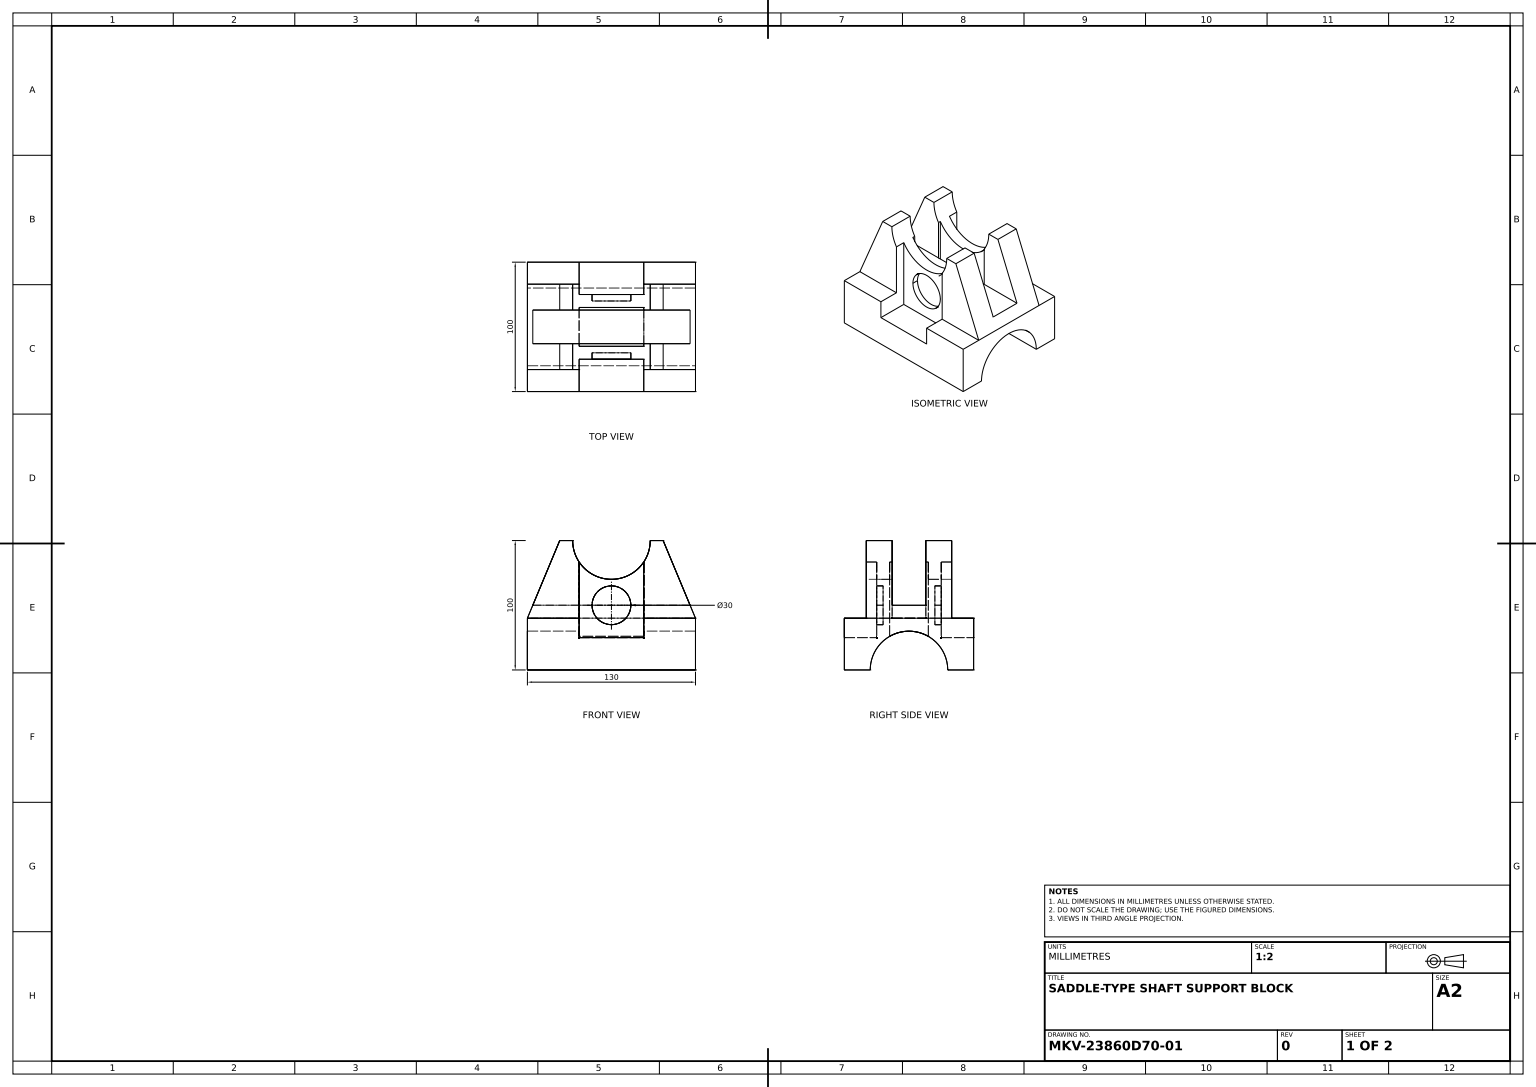
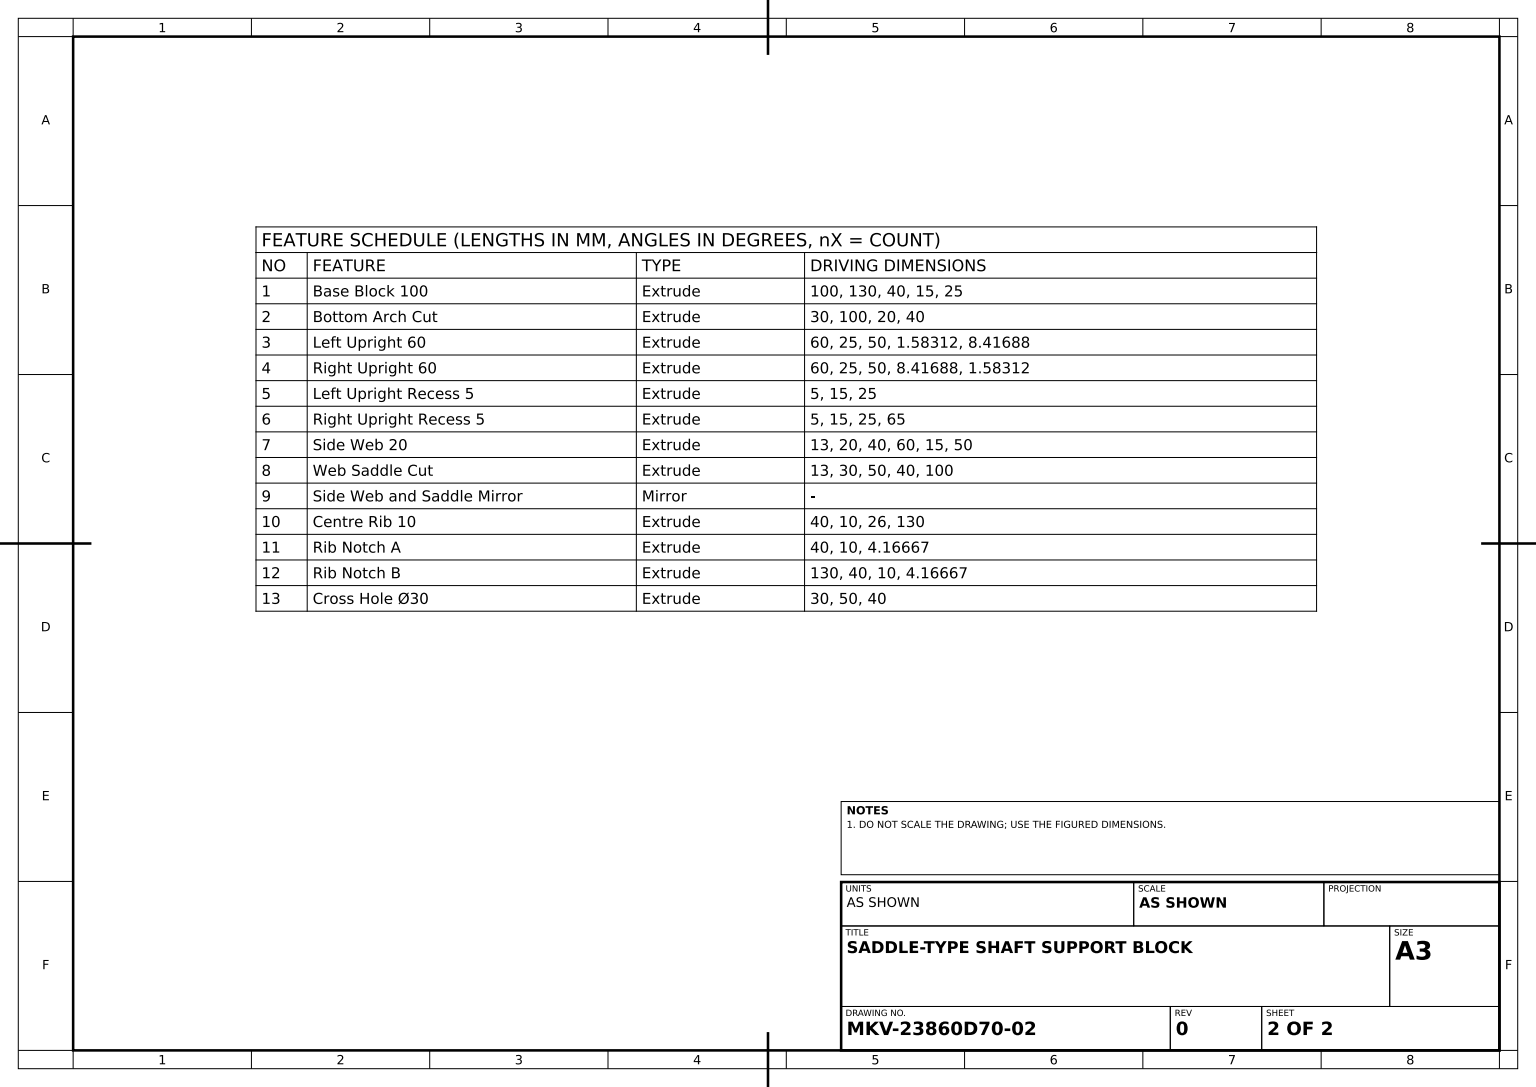
ISO-10303-21;
HEADER;
FILE_DESCRIPTION((''),'2;1');
FILE_NAME('','',(''),(''),'','','');
FILE_SCHEMA(('AUTOMOTIVE_DESIGN'));
ENDSEC;
DATA;
#1=APPLICATION_CONTEXT('');
#2=PRODUCT_CONTEXT('',#1,'mechanical');
#3=PRODUCT('','','',(#2));
#4=PRODUCT_DEFINITION_FORMATION('','',#3);
#5=PRODUCT_DEFINITION_CONTEXT('',#1,'design');
#6=PRODUCT_DEFINITION('','',#4,#5);
#7=PRODUCT_DEFINITION_SHAPE('','',#6);
#8=(LENGTH_UNIT()NAMED_UNIT(*)SI_UNIT(.MILLI.,.METRE.));
#9=(NAMED_UNIT(*)PLANE_ANGLE_UNIT()SI_UNIT($,.RADIAN.));
#10=(NAMED_UNIT(*)SI_UNIT($,.STERADIAN.)SOLID_ANGLE_UNIT());
#11=UNCERTAINTY_MEASURE_WITH_UNIT(LENGTH_MEASURE(1.E-05),#8,'distance_accuracy_value','');
#12=(GEOMETRIC_REPRESENTATION_CONTEXT(3)GLOBAL_UNCERTAINTY_ASSIGNED_CONTEXT((#11))GLOBAL_UNIT_ASSIGNED_CONTEXT((#8,#9,#10))REPRESENTATION_CONTEXT('',''));
#13=CARTESIAN_POINT('',(90.,40.,-33.));
#14=VERTEX_POINT('',#13);
#15=CARTESIAN_POINT('',(90.,40.,-50.));
#16=VERTEX_POINT('',#15);
#17=CARTESIAN_POINT('',(90.,40.,50.));
#18=DIRECTION('',(0.,0.,-1.));
#19=VECTOR('',#18,1000.);
#20=LINE('',#17,#19);
#21=EDGE_CURVE('',#14,#16,#20,.T.);
#22=ORIENTED_EDGE('',*,*,#21,.F.);
#23=CARTESIAN_POINT('',(130.,40.,-33.));
#24=VERTEX_POINT('',#23);
#25=DIRECTION('',(1.,0.,0.));
#26=VECTOR('',#25,1000.);
#27=LINE('',#23,#26);
#28=EDGE_CURVE('',#14,#24,#27,.T.);
#29=ORIENTED_EDGE('',*,*,#28,.T.);
#30=CARTESIAN_POINT('',(130.,40.,-50.));
#31=VERTEX_POINT('',#30);
#32=CARTESIAN_POINT('',(130.,40.,50.));
#33=LINE('',#32,#19);
#34=EDGE_CURVE('',#24,#31,#33,.T.);
#35=ORIENTED_EDGE('',*,*,#34,.T.);
#36=CARTESIAN_POINT('',(0.,40.,-50.));
#37=DIRECTION('',(-1.,0.,0.));
#38=VECTOR('',#37,1000.);
#39=LINE('',#36,#38);
#40=EDGE_CURVE('',#31,#16,#39,.T.);
#41=ORIENTED_EDGE('',*,*,#40,.T.);
#42=EDGE_LOOP('',(#22,#29,#35,#41));
#43=FACE_OUTER_BOUND('',#42,.T.);
#44=CARTESIAN_POINT('',(0.,40.,50.));
#45=DIRECTION('',(0.,-1.,0.));
#46=AXIS2_PLACEMENT_3D('',#44,#45,#18);
#47=PLANE('',#46);
#48=ADVANCED_FACE('',(#43),#47,.F.);
#49=CARTESIAN_POINT('',(40.,83.416876,-15.));
#50=VERTEX_POINT('',#49);
#51=CARTESIAN_POINT('',(40.,25.980762,-15.));
#52=VERTEX_POINT('',#51);
#53=CARTESIAN_POINT('',(40.,85.,-15.));
#54=VECTOR('',#45,1000.);
#55=LINE('',#53,#54);
#56=EDGE_CURVE('',#50,#52,#55,.T.);
#57=ORIENTED_EDGE('',*,*,#56,.T.);
#58=CARTESIAN_POINT('',(90.,25.980762,-15.));
#59=VERTEX_POINT('',#58);
#60=CARTESIAN_POINT('',(0.,25.980762,-15.));
#61=LINE('',#60,#38);
#62=EDGE_CURVE('',#59,#52,#61,.T.);
#63=ORIENTED_EDGE('',*,*,#62,.F.);
#64=CARTESIAN_POINT('',(90.,83.416876,-15.));
#65=VERTEX_POINT('',#64);
#66=CARTESIAN_POINT('',(90.,85.,-15.));
#67=LINE('',#66,#54);
#68=EDGE_CURVE('',#65,#59,#67,.T.);
#69=ORIENTED_EDGE('',*,*,#68,.F.);
#70=CARTESIAN_POINT('',(65.,100.,-15.));
#71=DIRECTION('',(0.,0.,1.));
#72=AXIS2_PLACEMENT_3D('',#70,#71,#25);
#73=CIRCLE('',#72,30.);
#74=EDGE_CURVE('',#50,#65,#73,.T.);
#75=ORIENTED_EDGE('',*,*,#74,.F.);
#76=EDGE_LOOP('',(#57,#63,#69,#75));
#77=FACE_OUTER_BOUND('',#76,.T.);
#78=AXIS2_PLACEMENT_3D('',#66,#71,#25);
#79=PLANE('',#78);
#80=ADVANCED_FACE('',(#77),#79,.T.);
#81=CARTESIAN_POINT('',(50.,50.,25.));
#82=VERTEX_POINT('',#81);
#83=CARTESIAN_POINT('',(80.,50.,25.));
#84=VERTEX_POINT('',#83);
#85=CARTESIAN_POINT('',(65.,50.,25.));
#86=AXIS2_PLACEMENT_3D('',#85,#71,#25);
#87=CIRCLE('',#86,15.);
#88=EDGE_CURVE('',#82,#84,#87,.T.);
#89=ORIENTED_EDGE('',*,*,#88,.T.);
#90=CARTESIAN_POINT('',(80.,50.,20.));
#91=VERTEX_POINT('',#90);
#92=VECTOR('',#71,1000.);
#93=LINE('',#90,#92);
#94=EDGE_CURVE('',#91,#84,#93,.T.);
#95=ORIENTED_EDGE('',*,*,#94,.F.);
#96=CARTESIAN_POINT('',(50.,50.,20.));
#97=VERTEX_POINT('',#96);
#98=CARTESIAN_POINT('',(65.,50.,20.));
#99=AXIS2_PLACEMENT_3D('',#98,#71,#25);
#100=CIRCLE('',#99,15.);
#101=EDGE_CURVE('',#97,#91,#100,.T.);
#102=ORIENTED_EDGE('',*,*,#101,.F.);
#103=LINE('',#96,#92);
#104=EDGE_CURVE('',#97,#82,#103,.T.);
#105=ORIENTED_EDGE('',*,*,#104,.T.);
#106=EDGE_LOOP('',(#89,#95,#102,#105));
#107=FACE_OUTER_BOUND('',#106,.T.);
#108=CYLINDRICAL_SURFACE('',#99,15.);
#109=ADVANCED_FACE('',(#107),#108,.F.);
#110=CARTESIAN_POINT('',(90.,40.,13.));
#111=VERTEX_POINT('',#110);
#112=CARTESIAN_POINT('',(90.,40.,-13.));
#113=VERTEX_POINT('',#112);
#114=EDGE_CURVE('',#111,#113,#20,.T.);
#115=ORIENTED_EDGE('',*,*,#114,.F.);
#116=CARTESIAN_POINT('',(40.,40.,13.));
#117=VERTEX_POINT('',#116);
#118=CARTESIAN_POINT('',(0.,40.,13.));
#119=LINE('',#118,#26);
#120=EDGE_CURVE('',#117,#111,#119,.T.);
#121=ORIENTED_EDGE('',*,*,#120,.F.);
#122=CARTESIAN_POINT('',(40.,40.,-13.));
#123=VERTEX_POINT('',#122);
#124=CARTESIAN_POINT('',(40.,40.,50.));
#125=LINE('',#124,#19);
#126=EDGE_CURVE('',#117,#123,#125,.T.);
#127=ORIENTED_EDGE('',*,*,#126,.T.);
#128=CARTESIAN_POINT('',(130.,40.,-13.));
#129=LINE('',#128,#38);
#130=EDGE_CURVE('',#113,#123,#129,.T.);
#131=ORIENTED_EDGE('',*,*,#130,.F.);
#132=EDGE_LOOP('',(#115,#121,#127,#131));
#133=FACE_OUTER_BOUND('',#132,.T.);
#134=CARTESIAN_POINT('',(0.,40.,0.));
#135=DIRECTION('',(0.,1.,0.));
#136=AXIS2_PLACEMENT_3D('',#134,#135,#71);
#137=PLANE('',#136);
#138=ADVANCED_FACE('',(#133),#137,.F.);
#139=CARTESIAN_POINT('',(0.,40.,-33.));
#140=VERTEX_POINT('',#139);
#141=CARTESIAN_POINT('',(40.,40.,-33.));
#142=VERTEX_POINT('',#141);
#143=LINE('',#139,#26);
#144=EDGE_CURVE('',#140,#142,#143,.T.);
#145=ORIENTED_EDGE('',*,*,#144,.F.);
#146=CARTESIAN_POINT('',(25.,100.,-33.));
#147=VERTEX_POINT('',#146);
#148=DIRECTION('',(-0.384615385,-0.923076923,0.));
#149=VECTOR('',#148,1000.);
#150=LINE('',#146,#149);
#151=EDGE_CURVE('',#147,#140,#150,.T.);
#152=ORIENTED_EDGE('',*,*,#151,.F.);
#153=CARTESIAN_POINT('',(35.,100.,-33.));
#154=VERTEX_POINT('',#153);
#155=LINE('',#146,#38);
#156=EDGE_CURVE('',#154,#147,#155,.T.);
#157=ORIENTED_EDGE('',*,*,#156,.F.);
#158=CARTESIAN_POINT('',(40.,83.416876,-33.));
#159=VERTEX_POINT('',#158);
#160=CARTESIAN_POINT('',(65.,100.,-33.));
#161=AXIS2_PLACEMENT_3D('',#160,#71,#37);
#162=CIRCLE('',#161,30.);
#163=EDGE_CURVE('',#154,#159,#162,.T.);
#164=ORIENTED_EDGE('',*,*,#163,.T.);
#165=VECTOR('',#135,1000.);
#166=LINE('',#141,#165);
#167=EDGE_CURVE('',#142,#159,#166,.T.);
#168=ORIENTED_EDGE('',*,*,#167,.F.);
#169=EDGE_LOOP('',(#145,#152,#157,#164,#168));
#170=FACE_OUTER_BOUND('',#169,.T.);
#171=CARTESIAN_POINT('',(0.,0.,-33.));
#172=AXIS2_PLACEMENT_3D('',#171,#18,#25);
#173=PLANE('',#172);
#174=ADVANCED_FACE('',(#170),#173,.T.);
#175=CARTESIAN_POINT('',(80.,50.,-20.));
#176=VERTEX_POINT('',#175);
#177=CARTESIAN_POINT('',(50.,50.,-20.));
#178=VERTEX_POINT('',#177);
#179=CARTESIAN_POINT('',(65.,50.,-20.));
#180=AXIS2_PLACEMENT_3D('',#179,#18,#37);
#181=CIRCLE('',#180,15.);
#182=EDGE_CURVE('',#176,#178,#181,.T.);
#183=ORIENTED_EDGE('',*,*,#182,.F.);
#184=CARTESIAN_POINT('',(80.,50.,-25.));
#185=VERTEX_POINT('',#184);
#186=LINE('',#175,#19);
#187=EDGE_CURVE('',#176,#185,#186,.T.);
#188=ORIENTED_EDGE('',*,*,#187,.T.);
#189=CARTESIAN_POINT('',(50.,50.,-25.));
#190=VERTEX_POINT('',#189);
#191=CARTESIAN_POINT('',(65.,50.,-25.));
#192=AXIS2_PLACEMENT_3D('',#191,#18,#37);
#193=CIRCLE('',#192,15.);
#194=EDGE_CURVE('',#185,#190,#193,.T.);
#195=ORIENTED_EDGE('',*,*,#194,.T.);
#196=LINE('',#177,#19);
#197=EDGE_CURVE('',#178,#190,#196,.T.);
#198=ORIENTED_EDGE('',*,*,#197,.F.);
#199=EDGE_LOOP('',(#183,#188,#195,#198));
#200=FACE_OUTER_BOUND('',#199,.T.);
#201=CYLINDRICAL_SURFACE('',#180,15.);
#202=ADVANCED_FACE('',(#200),#201,.F.);
#203=CARTESIAN_POINT('',(35.,100.,33.));
#204=VERTEX_POINT('',#203);
#205=CARTESIAN_POINT('',(35.,100.,13.));
#206=VERTEX_POINT('',#205);
#207=CARTESIAN_POINT('',(35.,100.,-50.));
#208=LINE('',#207,#19);
#209=EDGE_CURVE('',#204,#206,#208,.T.);
#210=ORIENTED_EDGE('',*,*,#209,.F.);
#211=CARTESIAN_POINT('',(40.,83.416876,33.));
#212=VERTEX_POINT('',#211);
#213=CARTESIAN_POINT('',(65.,100.,33.));
#214=AXIS2_PLACEMENT_3D('',#213,#71,#25);
#215=CIRCLE('',#214,30.);
#216=EDGE_CURVE('',#204,#212,#215,.T.);
#217=ORIENTED_EDGE('',*,*,#216,.T.);
#218=CARTESIAN_POINT('',(40.,83.416876,25.));
#219=VERTEX_POINT('',#218);
#220=CARTESIAN_POINT('',(40.,83.416876,-50.));
#221=LINE('',#220,#92);
#222=EDGE_CURVE('',#219,#212,#221,.T.);
#223=ORIENTED_EDGE('',*,*,#222,.F.);
#224=CARTESIAN_POINT('',(90.,83.416876,25.));
#225=VERTEX_POINT('',#224);
#226=CARTESIAN_POINT('',(65.,100.,25.));
#227=AXIS2_PLACEMENT_3D('',#226,#18,#37);
#228=CIRCLE('',#227,30.);
#229=EDGE_CURVE('',#225,#219,#228,.T.);
#230=ORIENTED_EDGE('',*,*,#229,.F.);
#231=CARTESIAN_POINT('',(90.,83.416876,33.));
#232=VERTEX_POINT('',#231);
#233=CARTESIAN_POINT('',(90.,83.416876,-50.));
#234=LINE('',#233,#19);
#235=EDGE_CURVE('',#232,#225,#234,.T.);
#236=ORIENTED_EDGE('',*,*,#235,.F.);
#237=CARTESIAN_POINT('',(95.,100.,33.));
#238=VERTEX_POINT('',#237);
#239=AXIS2_PLACEMENT_3D('',#213,#18,#37);
#240=CIRCLE('',#239,30.);
#241=EDGE_CURVE('',#238,#232,#240,.T.);
#242=ORIENTED_EDGE('',*,*,#241,.F.);
#243=CARTESIAN_POINT('',(95.,100.,13.));
#244=VERTEX_POINT('',#243);
#245=CARTESIAN_POINT('',(95.,100.,-50.));
#246=LINE('',#245,#92);
#247=EDGE_CURVE('',#244,#238,#246,.T.);
#248=ORIENTED_EDGE('',*,*,#247,.F.);
#249=CARTESIAN_POINT('',(90.,83.416876,13.));
#250=VERTEX_POINT('',#249);
#251=CARTESIAN_POINT('',(65.,100.,13.));
#252=AXIS2_PLACEMENT_3D('',#251,#18,#37);
#253=CIRCLE('',#252,30.);
#254=EDGE_CURVE('',#244,#250,#253,.T.);
#255=ORIENTED_EDGE('',*,*,#254,.T.);
#256=CARTESIAN_POINT('',(90.,83.416876,15.));
#257=VERTEX_POINT('',#256);
#258=EDGE_CURVE('',#257,#250,#234,.T.);
#259=ORIENTED_EDGE('',*,*,#258,.F.);
#260=CARTESIAN_POINT('',(40.,83.416876,15.));
#261=VERTEX_POINT('',#260);
#262=CARTESIAN_POINT('',(65.,100.,15.));
#263=AXIS2_PLACEMENT_3D('',#262,#71,#25);
#264=CIRCLE('',#263,30.);
#265=EDGE_CURVE('',#261,#257,#264,.T.);
#266=ORIENTED_EDGE('',*,*,#265,.F.);
#267=CARTESIAN_POINT('',(40.,83.416876,13.));
#268=VERTEX_POINT('',#267);
#269=EDGE_CURVE('',#268,#261,#221,.T.);
#270=ORIENTED_EDGE('',*,*,#269,.F.);
#271=AXIS2_PLACEMENT_3D('',#251,#71,#25);
#272=CIRCLE('',#271,30.);
#273=EDGE_CURVE('',#206,#268,#272,.T.);
#274=ORIENTED_EDGE('',*,*,#273,.F.);
#275=EDGE_LOOP('',(#210,#217,#223,#230,#236,#242,#248,#255,#259,#266,#270,#274));
#276=FACE_OUTER_BOUND('',#275,.T.);
#277=CARTESIAN_POINT('',(65.,100.,-50.));
#278=AXIS2_PLACEMENT_3D('',#277,#71,#25);
#279=CYLINDRICAL_SURFACE('',#278,30.);
#280=ADVANCED_FACE('',(#276),#279,.F.);
#281=CARTESIAN_POINT('',(40.,40.,33.));
#282=VERTEX_POINT('',#281);
#283=LINE('',#281,#165);
#284=EDGE_CURVE('',#282,#212,#283,.T.);
#285=ORIENTED_EDGE('',*,*,#284,.F.);
#286=VERTEX_POINT('',#124);
#287=EDGE_CURVE('',#286,#282,#125,.T.);
#288=ORIENTED_EDGE('',*,*,#287,.F.);
#289=CARTESIAN_POINT('',(40.,25.,50.));
#290=VERTEX_POINT('',#289);
#291=CARTESIAN_POINT('',(40.,0.,50.));
#292=LINE('',#291,#165);
#293=EDGE_CURVE('',#290,#286,#292,.T.);
#294=ORIENTED_EDGE('',*,*,#293,.F.);
#295=CARTESIAN_POINT('',(40.,25.,25.));
#296=VERTEX_POINT('',#295);
#297=LINE('',#289,#19);
#298=EDGE_CURVE('',#290,#296,#297,.T.);
#299=ORIENTED_EDGE('',*,*,#298,.T.);
#300=CARTESIAN_POINT('',(40.,85.,25.));
#301=LINE('',#300,#54);
#302=EDGE_CURVE('',#219,#296,#301,.T.);
#303=ORIENTED_EDGE('',*,*,#302,.F.);
#304=ORIENTED_EDGE('',*,*,#222,.T.);
#305=EDGE_LOOP('',(#285,#288,#294,#299,#303,#304));
#306=FACE_OUTER_BOUND('',#305,.T.);
#307=AXIS2_PLACEMENT_3D('',#291,#37,#71);
#308=PLANE('',#307);
#309=ADVANCED_FACE('',(#306),#308,.F.);
#310=CARTESIAN_POINT('',(40.,40.,-50.));
#311=VERTEX_POINT('',#310);
#312=EDGE_CURVE('',#142,#311,#125,.T.);
#313=ORIENTED_EDGE('',*,*,#312,.T.);
#314=VERTEX_POINT('',#36);
#315=EDGE_CURVE('',#311,#314,#39,.T.);
#316=ORIENTED_EDGE('',*,*,#315,.T.);
#317=LINE('',#44,#19);
#318=EDGE_CURVE('',#140,#314,#317,.T.);
#319=ORIENTED_EDGE('',*,*,#318,.F.);
#320=ORIENTED_EDGE('',*,*,#144,.T.);
#321=EDGE_LOOP('',(#313,#316,#319,#320));
#322=FACE_OUTER_BOUND('',#321,.T.);
#323=ADVANCED_FACE('',(#322),#47,.F.);
#324=CARTESIAN_POINT('',(90.,50.,13.));
#325=VERTEX_POINT('',#324);
#326=LINE('',#110,#54);
#327=EDGE_CURVE('',#325,#111,#326,.T.);
#328=ORIENTED_EDGE('',*,*,#327,.T.);
#329=ORIENTED_EDGE('',*,*,#114,.T.);
#330=CARTESIAN_POINT('',(90.,50.,-13.));
#331=VERTEX_POINT('',#330);
#332=LINE('',#112,#54);
#333=EDGE_CURVE('',#331,#113,#332,.T.);
#334=ORIENTED_EDGE('',*,*,#333,.F.);
#335=CARTESIAN_POINT('',(90.,83.416876,-13.));
#336=VERTEX_POINT('',#335);
#337=EDGE_CURVE('',#336,#331,#332,.T.);
#338=ORIENTED_EDGE('',*,*,#337,.F.);
#339=CARTESIAN_POINT('',(90.,83.416876,50.));
#340=LINE('',#339,#92);
#341=EDGE_CURVE('',#65,#336,#340,.T.);
#342=ORIENTED_EDGE('',*,*,#341,.F.);
#343=ORIENTED_EDGE('',*,*,#68,.T.);
#344=CARTESIAN_POINT('',(90.,25.980762,15.));
#345=VERTEX_POINT('',#344);
#346=CARTESIAN_POINT('',(90.,0.,0.));
#347=AXIS2_PLACEMENT_3D('',#346,#25,#18);
#348=CIRCLE('',#347,30.);
#349=EDGE_CURVE('',#59,#345,#348,.T.);
#350=ORIENTED_EDGE('',*,*,#349,.T.);
#351=CARTESIAN_POINT('',(90.,85.,15.));
#352=LINE('',#351,#54);
#353=EDGE_CURVE('',#257,#345,#352,.T.);
#354=ORIENTED_EDGE('',*,*,#353,.F.);
#355=ORIENTED_EDGE('',*,*,#258,.T.);
#356=EDGE_CURVE('',#250,#325,#326,.T.);
#357=ORIENTED_EDGE('',*,*,#356,.T.);
#358=EDGE_LOOP('',(#328,#329,#334,#338,#342,#343,#350,#354,#355,#357));
#359=FACE_OUTER_BOUND('',#358,.T.);
#360=CARTESIAN_POINT('',(90.,0.,50.));
#361=AXIS2_PLACEMENT_3D('',#360,#25,#18);
#362=PLANE('',#361);
#363=ADVANCED_FACE('',(#359),#362,.F.);
#364=CARTESIAN_POINT('',(125.833333,50.,13.));
#365=VERTEX_POINT('',#364);
#366=CARTESIAN_POINT('',(0.,50.,13.));
#367=LINE('',#366,#26);
#368=EDGE_CURVE('',#325,#365,#367,.T.);
#369=ORIENTED_EDGE('',*,*,#368,.F.);
#370=ORIENTED_EDGE('',*,*,#356,.F.);
#371=ORIENTED_EDGE('',*,*,#254,.F.);
#372=CARTESIAN_POINT('',(105.,100.,13.));
#373=VERTEX_POINT('',#372);
#374=CARTESIAN_POINT('',(90.,100.,13.));
#375=LINE('',#374,#38);
#376=EDGE_CURVE('',#373,#244,#375,.T.);
#377=ORIENTED_EDGE('',*,*,#376,.F.);
#378=CARTESIAN_POINT('',(130.,40.,13.));
#379=DIRECTION('',(-0.384615385,0.923076923,0.));
#380=VECTOR('',#379,1000.);
#381=LINE('',#378,#380);
#382=EDGE_CURVE('',#365,#373,#381,.T.);
#383=ORIENTED_EDGE('',*,*,#382,.F.);
#384=EDGE_LOOP('',(#369,#370,#371,#377,#383));
#385=FACE_OUTER_BOUND('',#384,.T.);
#386=CARTESIAN_POINT('',(0.,0.,13.));
#387=AXIS2_PLACEMENT_3D('',#386,#18,#37);
#388=PLANE('',#387);
#389=ADVANCED_FACE('',(#385),#388,.T.);
#390=ORIENTED_EDGE('',*,*,#337,.T.);
#391=CARTESIAN_POINT('',(125.833333,50.,-13.));
#392=VERTEX_POINT('',#391);
#393=CARTESIAN_POINT('',(0.,50.,-13.));
#394=LINE('',#393,#38);
#395=EDGE_CURVE('',#392,#331,#394,.T.);
#396=ORIENTED_EDGE('',*,*,#395,.F.);
#397=CARTESIAN_POINT('',(105.,100.,-13.));
#398=VERTEX_POINT('',#397);
#399=LINE('',#128,#380);
#400=EDGE_CURVE('',#392,#398,#399,.T.);
#401=ORIENTED_EDGE('',*,*,#400,.T.);
#402=CARTESIAN_POINT('',(95.,100.,-13.));
#403=VERTEX_POINT('',#402);
#404=CARTESIAN_POINT('',(90.,100.,-13.));
#405=LINE('',#404,#38);
#406=EDGE_CURVE('',#398,#403,#405,.T.);
#407=ORIENTED_EDGE('',*,*,#406,.T.);
#408=CARTESIAN_POINT('',(65.,100.,-13.));
#409=AXIS2_PLACEMENT_3D('',#408,#18,#25);
#410=CIRCLE('',#409,30.);
#411=EDGE_CURVE('',#403,#336,#410,.T.);
#412=ORIENTED_EDGE('',*,*,#411,.T.);
#413=EDGE_LOOP('',(#390,#396,#401,#407,#412));
#414=FACE_OUTER_BOUND('',#413,.T.);
#415=CARTESIAN_POINT('',(0.,0.,-13.));
#416=AXIS2_PLACEMENT_3D('',#415,#71,#37);
#417=PLANE('',#416);
#418=ADVANCED_FACE('',(#414),#417,.T.);
#419=ORIENTED_EDGE('',*,*,#287,.T.);
#420=CARTESIAN_POINT('',(0.,40.,33.));
#421=VERTEX_POINT('',#420);
#422=LINE('',#420,#26);
#423=EDGE_CURVE('',#421,#282,#422,.T.);
#424=ORIENTED_EDGE('',*,*,#423,.F.);
#425=VERTEX_POINT('',#44);
#426=EDGE_CURVE('',#425,#421,#317,.T.);
#427=ORIENTED_EDGE('',*,*,#426,.F.);
#428=LINE('',#44,#38);
#429=EDGE_CURVE('',#286,#425,#428,.T.);
#430=ORIENTED_EDGE('',*,*,#429,.F.);
#431=EDGE_LOOP('',(#419,#424,#427,#430));
#432=FACE_OUTER_BOUND('',#431,.T.);
#433=ADVANCED_FACE('',(#432),#47,.F.);
#434=ORIENTED_EDGE('',*,*,#120,.T.);
#435=ORIENTED_EDGE('',*,*,#327,.F.);
#436=CARTESIAN_POINT('',(40.,50.,13.));
#437=VERTEX_POINT('',#436);
#438=EDGE_CURVE('',#437,#325,#367,.T.);
#439=ORIENTED_EDGE('',*,*,#438,.F.);
#440=LINE('',#116,#165);
#441=EDGE_CURVE('',#117,#437,#440,.T.);
#442=ORIENTED_EDGE('',*,*,#441,.F.);
#443=EDGE_LOOP('',(#434,#435,#439,#442));
#444=FACE_OUTER_BOUND('',#443,.T.);
#445=AXIS2_PLACEMENT_3D('',#366,#18,#37);
#446=PLANE('',#445);
#447=ADVANCED_FACE('',(#444),#446,.F.);
#448=CARTESIAN_POINT('',(40.,50.,-13.));
#449=VERTEX_POINT('',#448);
#450=CARTESIAN_POINT('',(130.,50.,-13.));
#451=LINE('',#450,#38);
#452=EDGE_CURVE('',#331,#449,#451,.T.);
#453=ORIENTED_EDGE('',*,*,#452,.F.);
#454=ORIENTED_EDGE('',*,*,#333,.T.);
#455=ORIENTED_EDGE('',*,*,#130,.T.);
#456=LINE('',#122,#165);
#457=EDGE_CURVE('',#123,#449,#456,.T.);
#458=ORIENTED_EDGE('',*,*,#457,.T.);
#459=EDGE_LOOP('',(#453,#454,#455,#458));
#460=FACE_OUTER_BOUND('',#459,.T.);
#461=AXIS2_PLACEMENT_3D('',#450,#71,#25);
#462=PLANE('',#461);
#463=ADVANCED_FACE('',(#460),#462,.F.);
#464=VERTEX_POINT('',#17);
#465=CARTESIAN_POINT('',(90.,40.,33.));
#466=VERTEX_POINT('',#465);
#467=EDGE_CURVE('',#464,#466,#20,.T.);
#468=ORIENTED_EDGE('',*,*,#467,.T.);
#469=LINE('',#465,#54);
#470=EDGE_CURVE('',#232,#466,#469,.T.);
#471=ORIENTED_EDGE('',*,*,#470,.F.);
#472=ORIENTED_EDGE('',*,*,#235,.T.);
#473=CARTESIAN_POINT('',(90.,25.,25.));
#474=VERTEX_POINT('',#473);
#475=CARTESIAN_POINT('',(90.,85.,25.));
#476=LINE('',#475,#54);
#477=EDGE_CURVE('',#225,#474,#476,.T.);
#478=ORIENTED_EDGE('',*,*,#477,.T.);
#479=CARTESIAN_POINT('',(90.,25.,50.));
#480=VERTEX_POINT('',#479);
#481=LINE('',#479,#19);
#482=EDGE_CURVE('',#480,#474,#481,.T.);
#483=ORIENTED_EDGE('',*,*,#482,.F.);
#484=LINE('',#360,#54);
#485=EDGE_CURVE('',#464,#480,#484,.T.);
#486=ORIENTED_EDGE('',*,*,#485,.F.);
#487=EDGE_LOOP('',(#468,#471,#472,#478,#483,#486));
#488=FACE_OUTER_BOUND('',#487,.T.);
#489=ADVANCED_FACE('',(#488),#362,.F.);
#490=CARTESIAN_POINT('',(4.166667,50.,13.));
#491=VERTEX_POINT('',#490);
#492=CARTESIAN_POINT('',(4.166667,50.,-13.));
#493=VERTEX_POINT('',#492);
#494=CARTESIAN_POINT('',(4.166667,50.,0.));
#495=LINE('',#494,#19);
#496=EDGE_CURVE('',#491,#493,#495,.T.);
#497=ORIENTED_EDGE('',*,*,#496,.T.);
#498=CARTESIAN_POINT('',(25.,100.,-13.));
#499=VERTEX_POINT('',#498);
#500=LINE('',#498,#149);
#501=EDGE_CURVE('',#499,#493,#500,.T.);
#502=ORIENTED_EDGE('',*,*,#501,.F.);
#503=LINE('',#146,#92);
#504=EDGE_CURVE('',#147,#499,#503,.T.);
#505=ORIENTED_EDGE('',*,*,#504,.F.);
#506=ORIENTED_EDGE('',*,*,#151,.T.);
#507=LINE('',#420,#19);
#508=EDGE_CURVE('',#421,#140,#507,.T.);
#509=ORIENTED_EDGE('',*,*,#508,.F.);
#510=CARTESIAN_POINT('',(25.,100.,33.));
#511=VERTEX_POINT('',#510);
#512=LINE('',#510,#149);
#513=EDGE_CURVE('',#511,#421,#512,.T.);
#514=ORIENTED_EDGE('',*,*,#513,.F.);
#515=CARTESIAN_POINT('',(25.,100.,13.));
#516=VERTEX_POINT('',#515);
#517=LINE('',#510,#19);
#518=EDGE_CURVE('',#511,#516,#517,.T.);
#519=ORIENTED_EDGE('',*,*,#518,.T.);
#520=LINE('',#515,#149);
#521=EDGE_CURVE('',#516,#491,#520,.T.);
#522=ORIENTED_EDGE('',*,*,#521,.T.);
#523=EDGE_LOOP('',(#497,#502,#505,#506,#509,#514,#519,#522));
#524=FACE_OUTER_BOUND('',#523,.T.);
#525=DIRECTION('',(0.923076923,-0.384615385,0.));
#526=DIRECTION('',(0.384615385,0.923076923,0.));
#527=AXIS2_PLACEMENT_3D('',#510,#525,#526);
#528=PLANE('',#527);
#529=ADVANCED_FACE('',(#524),#528,.F.);
#530=CARTESIAN_POINT('',(105.,100.,33.));
#531=VERTEX_POINT('',#530);
#532=LINE('',#530,#19);
#533=EDGE_CURVE('',#531,#373,#532,.T.);
#534=ORIENTED_EDGE('',*,*,#533,.T.);
#535=ORIENTED_EDGE('',*,*,#376,.T.);
#536=ORIENTED_EDGE('',*,*,#247,.T.);
#537=CARTESIAN_POINT('',(90.,100.,33.));
#538=LINE('',#537,#38);
#539=EDGE_CURVE('',#531,#238,#538,.T.);
#540=ORIENTED_EDGE('',*,*,#539,.F.);
#541=EDGE_LOOP('',(#534,#535,#536,#540));
#542=FACE_OUTER_BOUND('',#541,.T.);
#543=AXIS2_PLACEMENT_3D('',#537,#45,#18);
#544=PLANE('',#543);
#545=ADVANCED_FACE('',(#542),#544,.F.);
#546=CARTESIAN_POINT('',(40.,25.980762,15.));
#547=VERTEX_POINT('',#546);
#548=CARTESIAN_POINT('',(40.,0.,0.));
#549=AXIS2_PLACEMENT_3D('',#548,#37,#71);
#550=CIRCLE('',#549,30.);
#551=EDGE_CURVE('',#547,#52,#550,.T.);
#552=ORIENTED_EDGE('',*,*,#551,.T.);
#553=ORIENTED_EDGE('',*,*,#56,.F.);
#554=CARTESIAN_POINT('',(40.,83.416876,-13.));
#555=VERTEX_POINT('',#554);
#556=CARTESIAN_POINT('',(40.,83.416876,50.));
#557=LINE('',#556,#19);
#558=EDGE_CURVE('',#555,#50,#557,.T.);
#559=ORIENTED_EDGE('',*,*,#558,.F.);
#560=EDGE_CURVE('',#449,#555,#456,.T.);
#561=ORIENTED_EDGE('',*,*,#560,.F.);
#562=ORIENTED_EDGE('',*,*,#457,.F.);
#563=ORIENTED_EDGE('',*,*,#126,.F.);
#564=ORIENTED_EDGE('',*,*,#441,.T.);
#565=EDGE_CURVE('',#437,#268,#440,.T.);
#566=ORIENTED_EDGE('',*,*,#565,.T.);
#567=ORIENTED_EDGE('',*,*,#269,.T.);
#568=CARTESIAN_POINT('',(40.,85.,15.));
#569=LINE('',#568,#54);
#570=EDGE_CURVE('',#261,#547,#569,.T.);
#571=ORIENTED_EDGE('',*,*,#570,.T.);
#572=EDGE_LOOP('',(#552,#553,#559,#561,#562,#563,#564,#566,#567,#571));
#573=FACE_OUTER_BOUND('',#572,.T.);
#574=ADVANCED_FACE('',(#573),#308,.F.);
#575=CARTESIAN_POINT('',(0.,0.,50.));
#576=VERTEX_POINT('',#575);
#577=CARTESIAN_POINT('',(130.,0.,50.));
#578=VERTEX_POINT('',#577);
#579=LINE('',#575,#26);
#580=EDGE_CURVE('',#576,#578,#579,.T.);
#581=ORIENTED_EDGE('',*,*,#580,.F.);
#582=CARTESIAN_POINT('',(0.,0.,30.));
#583=VERTEX_POINT('',#582);
#584=LINE('',#575,#19);
#585=EDGE_CURVE('',#576,#583,#584,.T.);
#586=ORIENTED_EDGE('',*,*,#585,.T.);
#587=CARTESIAN_POINT('',(130.,0.,30.));
#588=VERTEX_POINT('',#587);
#589=LINE('',#582,#26);
#590=EDGE_CURVE('',#583,#588,#589,.T.);
#591=ORIENTED_EDGE('',*,*,#590,.T.);
#592=LINE('',#577,#19);
#593=EDGE_CURVE('',#578,#588,#592,.T.);
#594=ORIENTED_EDGE('',*,*,#593,.F.);
#595=EDGE_LOOP('',(#581,#586,#591,#594));
#596=FACE_OUTER_BOUND('',#595,.T.);
#597=AXIS2_PLACEMENT_3D('',#575,#135,#71);
#598=PLANE('',#597);
#599=ADVANCED_FACE('',(#596),#598,.F.);
#600=ORIENTED_EDGE('',*,*,#265,.T.);
#601=ORIENTED_EDGE('',*,*,#353,.T.);
#602=CARTESIAN_POINT('',(0.,25.980762,15.));
#603=LINE('',#602,#38);
#604=EDGE_CURVE('',#345,#547,#603,.T.);
#605=ORIENTED_EDGE('',*,*,#604,.T.);
#606=ORIENTED_EDGE('',*,*,#570,.F.);
#607=EDGE_LOOP('',(#600,#601,#605,#606));
#608=FACE_OUTER_BOUND('',#607,.T.);
#609=CARTESIAN_POINT('',(0.,85.,15.));
#610=AXIS2_PLACEMENT_3D('',#609,#71,#25);
#611=PLANE('',#610);
#612=ADVANCED_FACE('',(#608),#611,.F.);
#613=CARTESIAN_POINT('',(0.,0.,-50.));
#614=VERTEX_POINT('',#613);
#615=CARTESIAN_POINT('',(130.,0.,-50.));
#616=VERTEX_POINT('',#615);
#617=LINE('',#613,#26);
#618=EDGE_CURVE('',#614,#616,#617,.T.);
#619=ORIENTED_EDGE('',*,*,#618,.T.);
#620=CARTESIAN_POINT('',(130.,0.,-30.));
#621=VERTEX_POINT('',#620);
#622=EDGE_CURVE('',#621,#616,#592,.T.);
#623=ORIENTED_EDGE('',*,*,#622,.F.);
#624=CARTESIAN_POINT('',(0.,0.,-30.));
#625=VERTEX_POINT('',#624);
#626=LINE('',#624,#38);
#627=EDGE_CURVE('',#621,#625,#626,.T.);
#628=ORIENTED_EDGE('',*,*,#627,.T.);
#629=EDGE_CURVE('',#625,#614,#584,.T.);
#630=ORIENTED_EDGE('',*,*,#629,.T.);
#631=EDGE_LOOP('',(#619,#623,#628,#630));
#632=FACE_OUTER_BOUND('',#631,.T.);
#633=ADVANCED_FACE('',(#632),#598,.F.);
#634=CARTESIAN_POINT('',(95.,100.,-33.));
#635=VERTEX_POINT('',#634);
#636=CARTESIAN_POINT('',(90.,83.416876,-33.));
#637=VERTEX_POINT('',#636);
#638=AXIS2_PLACEMENT_3D('',#160,#18,#25);
#639=CIRCLE('',#638,30.);
#640=EDGE_CURVE('',#635,#637,#639,.T.);
#641=ORIENTED_EDGE('',*,*,#640,.T.);
#642=CARTESIAN_POINT('',(90.,83.416876,-25.));
#643=VERTEX_POINT('',#642);
#644=EDGE_CURVE('',#637,#643,#340,.T.);
#645=ORIENTED_EDGE('',*,*,#644,.T.);
#646=CARTESIAN_POINT('',(40.,83.416876,-25.));
#647=VERTEX_POINT('',#646);
#648=CARTESIAN_POINT('',(65.,100.,-25.));
#649=AXIS2_PLACEMENT_3D('',#648,#18,#37);
#650=CIRCLE('',#649,30.);
#651=EDGE_CURVE('',#643,#647,#650,.T.);
#652=ORIENTED_EDGE('',*,*,#651,.T.);
#653=EDGE_CURVE('',#647,#159,#557,.T.);
#654=ORIENTED_EDGE('',*,*,#653,.T.);
#655=ORIENTED_EDGE('',*,*,#163,.F.);
#656=CARTESIAN_POINT('',(35.,100.,-13.));
#657=VERTEX_POINT('',#656);
#658=CARTESIAN_POINT('',(35.,100.,50.));
#659=LINE('',#658,#19);
#660=EDGE_CURVE('',#657,#154,#659,.T.);
#661=ORIENTED_EDGE('',*,*,#660,.F.);
#662=AXIS2_PLACEMENT_3D('',#408,#71,#37);
#663=CIRCLE('',#662,30.);
#664=EDGE_CURVE('',#657,#555,#663,.T.);
#665=ORIENTED_EDGE('',*,*,#664,.T.);
#666=ORIENTED_EDGE('',*,*,#558,.T.);
#667=ORIENTED_EDGE('',*,*,#74,.T.);
#668=ORIENTED_EDGE('',*,*,#341,.T.);
#669=ORIENTED_EDGE('',*,*,#411,.F.);
#670=CARTESIAN_POINT('',(95.,100.,50.));
#671=LINE('',#670,#92);
#672=EDGE_CURVE('',#635,#403,#671,.T.);
#673=ORIENTED_EDGE('',*,*,#672,.F.);
#674=EDGE_LOOP('',(#641,#645,#652,#654,#655,#661,#665,#666,#667,#668,#669,#673));
#675=FACE_OUTER_BOUND('',#674,.T.);
#676=ADVANCED_FACE('',(#675),#279,.F.);
#677=ORIENTED_EDGE('',*,*,#182,.T.);
#678=EDGE_CURVE('',#178,#176,#181,.T.);
#679=ORIENTED_EDGE('',*,*,#678,.T.);
#680=EDGE_LOOP('',(#677,#679));
#681=FACE_OUTER_BOUND('',#680,.T.);
#682=PLANE('',#180);
#683=ADVANCED_FACE('',(#681),#682,.T.);
#684=VERTEX_POINT('',#32);
#685=CARTESIAN_POINT('',(130.,40.,33.));
#686=VERTEX_POINT('',#685);
#687=EDGE_CURVE('',#684,#686,#33,.T.);
#688=ORIENTED_EDGE('',*,*,#687,.F.);
#689=LINE('',#577,#165);
#690=EDGE_CURVE('',#578,#684,#689,.T.);
#691=ORIENTED_EDGE('',*,*,#690,.F.);
#692=ORIENTED_EDGE('',*,*,#593,.T.);
#693=CARTESIAN_POINT('',(130.,0.,0.));
#694=AXIS2_PLACEMENT_3D('',#693,#25,#18);
#695=CIRCLE('',#694,30.);
#696=EDGE_CURVE('',#621,#588,#695,.T.);
#697=ORIENTED_EDGE('',*,*,#696,.F.);
#698=ORIENTED_EDGE('',*,*,#622,.T.);
#699=LINE('',#615,#165);
#700=EDGE_CURVE('',#616,#31,#699,.T.);
#701=ORIENTED_EDGE('',*,*,#700,.T.);
#702=ORIENTED_EDGE('',*,*,#34,.F.);
#703=LINE('',#685,#19);
#704=EDGE_CURVE('',#686,#24,#703,.T.);
#705=ORIENTED_EDGE('',*,*,#704,.F.);
#706=EDGE_LOOP('',(#688,#691,#692,#697,#698,#701,#702,#705));
#707=FACE_OUTER_BOUND('',#706,.T.);
#708=AXIS2_PLACEMENT_3D('',#577,#37,#71);
#709=PLANE('',#708);
#710=ADVANCED_FACE('',(#707),#709,.F.);
#711=ORIENTED_EDGE('',*,*,#560,.T.);
#712=ORIENTED_EDGE('',*,*,#664,.F.);
#713=LINE('',#498,#38);
#714=EDGE_CURVE('',#657,#499,#713,.T.);
#715=ORIENTED_EDGE('',*,*,#714,.T.);
#716=ORIENTED_EDGE('',*,*,#501,.T.);
#717=EDGE_CURVE('',#449,#493,#451,.T.);
#718=ORIENTED_EDGE('',*,*,#717,.F.);
#719=EDGE_LOOP('',(#711,#712,#715,#716,#718));
#720=FACE_OUTER_BOUND('',#719,.T.);
#721=AXIS2_PLACEMENT_3D('',#415,#18,#25);
#722=PLANE('',#721);
#723=ADVANCED_FACE('',(#720),#722,.F.);
#724=ORIENTED_EDGE('',*,*,#312,.F.);
#725=ORIENTED_EDGE('',*,*,#167,.T.);
#726=ORIENTED_EDGE('',*,*,#653,.F.);
#727=CARTESIAN_POINT('',(40.,25.,-25.));
#728=VERTEX_POINT('',#727);
#729=CARTESIAN_POINT('',(40.,85.,-25.));
#730=LINE('',#729,#54);
#731=EDGE_CURVE('',#647,#728,#730,.T.);
#732=ORIENTED_EDGE('',*,*,#731,.T.);
#733=CARTESIAN_POINT('',(40.,25.,-50.));
#734=VERTEX_POINT('',#733);
#735=EDGE_CURVE('',#728,#734,#297,.T.);
#736=ORIENTED_EDGE('',*,*,#735,.T.);
#737=CARTESIAN_POINT('',(40.,0.,-50.));
#738=LINE('',#737,#165);
#739=EDGE_CURVE('',#734,#311,#738,.T.);
#740=ORIENTED_EDGE('',*,*,#739,.T.);
#741=EDGE_LOOP('',(#724,#725,#726,#732,#736,#740));
#742=FACE_OUTER_BOUND('',#741,.T.);
#743=ADVANCED_FACE('',(#742),#308,.F.);
#744=ORIENTED_EDGE('',*,*,#704,.T.);
#745=CARTESIAN_POINT('',(105.,100.,-33.));
#746=VERTEX_POINT('',#745);
#747=LINE('',#23,#380);
#748=EDGE_CURVE('',#24,#746,#747,.T.);
#749=ORIENTED_EDGE('',*,*,#748,.T.);
#750=LINE('',#745,#92);
#751=EDGE_CURVE('',#746,#398,#750,.T.);
#752=ORIENTED_EDGE('',*,*,#751,.T.);
#753=ORIENTED_EDGE('',*,*,#400,.F.);
#754=CARTESIAN_POINT('',(125.833333,50.,0.));
#755=LINE('',#754,#92);
#756=EDGE_CURVE('',#392,#365,#755,.T.);
#757=ORIENTED_EDGE('',*,*,#756,.T.);
#758=ORIENTED_EDGE('',*,*,#382,.T.);
#759=ORIENTED_EDGE('',*,*,#533,.F.);
#760=LINE('',#685,#380);
#761=EDGE_CURVE('',#686,#531,#760,.T.);
#762=ORIENTED_EDGE('',*,*,#761,.F.);
#763=EDGE_LOOP('',(#744,#749,#752,#753,#757,#758,#759,#762));
#764=FACE_OUTER_BOUND('',#763,.T.);
#765=DIRECTION('',(-0.923076923,-0.384615385,0.));
#766=DIRECTION('',(0.384615385,-0.923076923,0.));
#767=AXIS2_PLACEMENT_3D('',#685,#765,#766);
#768=PLANE('',#767);
#769=ADVANCED_FACE('',(#764),#768,.F.);
#770=ORIENTED_EDGE('',*,*,#194,.F.);
#771=EDGE_CURVE('',#190,#185,#193,.T.);
#772=ORIENTED_EDGE('',*,*,#771,.F.);
#773=EDGE_LOOP('',(#770,#772));
#774=FACE_BOUND('',#773,.T.);
#775=ORIENTED_EDGE('',*,*,#731,.F.);
#776=ORIENTED_EDGE('',*,*,#651,.F.);
#777=CARTESIAN_POINT('',(90.,25.,-25.));
#778=VERTEX_POINT('',#777);
#779=CARTESIAN_POINT('',(90.,85.,-25.));
#780=LINE('',#779,#54);
#781=EDGE_CURVE('',#643,#778,#780,.T.);
#782=ORIENTED_EDGE('',*,*,#781,.T.);
#783=CARTESIAN_POINT('',(0.,25.,-25.));
#784=LINE('',#783,#26);
#785=EDGE_CURVE('',#728,#778,#784,.T.);
#786=ORIENTED_EDGE('',*,*,#785,.F.);
#787=EDGE_LOOP('',(#775,#776,#782,#786));
#788=FACE_OUTER_BOUND('',#787,.T.);
#789=CARTESIAN_POINT('',(0.,85.,-25.));
#790=AXIS2_PLACEMENT_3D('',#789,#18,#37);
#791=PLANE('',#790);
#792=ADVANCED_FACE('',(#774,#788),#791,.T.);
#793=LINE('',#13,#54);
#794=EDGE_CURVE('',#637,#14,#793,.T.);
#795=ORIENTED_EDGE('',*,*,#794,.F.);
#796=ORIENTED_EDGE('',*,*,#640,.F.);
#797=CARTESIAN_POINT('',(90.,100.,-33.));
#798=LINE('',#797,#38);
#799=EDGE_CURVE('',#746,#635,#798,.T.);
#800=ORIENTED_EDGE('',*,*,#799,.F.);
#801=ORIENTED_EDGE('',*,*,#748,.F.);
#802=ORIENTED_EDGE('',*,*,#28,.F.);
#803=EDGE_LOOP('',(#795,#796,#800,#801,#802));
#804=FACE_OUTER_BOUND('',#803,.T.);
#805=AXIS2_PLACEMENT_3D('',#171,#71,#37);
#806=PLANE('',#805);
#807=ADVANCED_FACE('',(#804),#806,.F.);
#808=ORIENTED_EDGE('',*,*,#423,.T.);
#809=ORIENTED_EDGE('',*,*,#284,.T.);
#810=ORIENTED_EDGE('',*,*,#216,.F.);
#811=LINE('',#510,#38);
#812=EDGE_CURVE('',#204,#511,#811,.T.);
#813=ORIENTED_EDGE('',*,*,#812,.T.);
#814=ORIENTED_EDGE('',*,*,#513,.T.);
#815=EDGE_LOOP('',(#808,#809,#810,#813,#814));
#816=FACE_OUTER_BOUND('',#815,.T.);
#817=CARTESIAN_POINT('',(0.,0.,33.));
#818=AXIS2_PLACEMENT_3D('',#817,#71,#25);
#819=PLANE('',#818);
#820=ADVANCED_FACE('',(#816),#819,.T.);
#821=CARTESIAN_POINT('',(0.,25.,50.));
#822=LINE('',#821,#26);
#823=EDGE_CURVE('',#290,#480,#822,.T.);
#824=ORIENTED_EDGE('',*,*,#823,.F.);
#825=ORIENTED_EDGE('',*,*,#293,.T.);
#826=ORIENTED_EDGE('',*,*,#429,.T.);
#827=LINE('',#575,#54);
#828=EDGE_CURVE('',#425,#576,#827,.T.);
#829=ORIENTED_EDGE('',*,*,#828,.T.);
#830=ORIENTED_EDGE('',*,*,#580,.T.);
#831=ORIENTED_EDGE('',*,*,#690,.T.);
#832=EDGE_CURVE('',#684,#464,#428,.T.);
#833=ORIENTED_EDGE('',*,*,#832,.T.);
#834=ORIENTED_EDGE('',*,*,#485,.T.);
#835=EDGE_LOOP('',(#824,#825,#826,#829,#830,#831,#833,#834));
#836=FACE_OUTER_BOUND('',#835,.T.);
#837=AXIS2_PLACEMENT_3D('',#575,#71,#25);
#838=PLANE('',#837);
#839=ADVANCED_FACE('',(#836),#838,.T.);
#840=ORIENTED_EDGE('',*,*,#315,.F.);
#841=ORIENTED_EDGE('',*,*,#739,.F.);
#842=CARTESIAN_POINT('',(90.,25.,-50.));
#843=VERTEX_POINT('',#842);
#844=CARTESIAN_POINT('',(0.,25.,-50.));
#845=LINE('',#844,#26);
#846=EDGE_CURVE('',#734,#843,#845,.T.);
#847=ORIENTED_EDGE('',*,*,#846,.T.);
#848=CARTESIAN_POINT('',(90.,0.,-50.));
#849=LINE('',#848,#54);
#850=EDGE_CURVE('',#16,#843,#849,.T.);
#851=ORIENTED_EDGE('',*,*,#850,.F.);
#852=ORIENTED_EDGE('',*,*,#40,.F.);
#853=ORIENTED_EDGE('',*,*,#700,.F.);
#854=ORIENTED_EDGE('',*,*,#618,.F.);
#855=LINE('',#613,#54);
#856=EDGE_CURVE('',#314,#614,#855,.T.);
#857=ORIENTED_EDGE('',*,*,#856,.F.);
#858=EDGE_LOOP('',(#840,#841,#847,#851,#852,#853,#854,#857));
#859=FACE_OUTER_BOUND('',#858,.T.);
#860=AXIS2_PLACEMENT_3D('',#613,#71,#25);
#861=PLANE('',#860);
#862=ADVANCED_FACE('',(#859),#861,.F.);
#863=ORIENTED_EDGE('',*,*,#241,.T.);
#864=ORIENTED_EDGE('',*,*,#470,.T.);
#865=LINE('',#685,#26);
#866=EDGE_CURVE('',#466,#686,#865,.T.);
#867=ORIENTED_EDGE('',*,*,#866,.T.);
#868=ORIENTED_EDGE('',*,*,#761,.T.);
#869=ORIENTED_EDGE('',*,*,#539,.T.);
#870=EDGE_LOOP('',(#863,#864,#867,#868,#869));
#871=FACE_OUTER_BOUND('',#870,.T.);
#872=AXIS2_PLACEMENT_3D('',#817,#18,#37);
#873=PLANE('',#872);
#874=ADVANCED_FACE('',(#871),#873,.F.);
#875=ORIENTED_EDGE('',*,*,#302,.T.);
#876=CARTESIAN_POINT('',(0.,25.,25.));
#877=LINE('',#876,#26);
#878=EDGE_CURVE('',#296,#474,#877,.T.);
#879=ORIENTED_EDGE('',*,*,#878,.T.);
#880=ORIENTED_EDGE('',*,*,#477,.F.);
#881=ORIENTED_EDGE('',*,*,#229,.T.);
#882=EDGE_LOOP('',(#875,#879,#880,#881));
#883=FACE_OUTER_BOUND('',#882,.T.);
#884=EDGE_CURVE('',#84,#82,#87,.T.);
#885=ORIENTED_EDGE('',*,*,#884,.F.);
#886=ORIENTED_EDGE('',*,*,#88,.F.);
#887=EDGE_LOOP('',(#885,#886));
#888=FACE_BOUND('',#887,.T.);
#889=CARTESIAN_POINT('',(0.,85.,25.));
#890=AXIS2_PLACEMENT_3D('',#889,#18,#37);
#891=PLANE('',#890);
#892=ADVANCED_FACE('',(#883,#888),#891,.F.);
#893=ORIENTED_EDGE('',*,*,#585,.F.);
#894=ORIENTED_EDGE('',*,*,#828,.F.);
#895=ORIENTED_EDGE('',*,*,#426,.T.);
#896=ORIENTED_EDGE('',*,*,#508,.T.);
#897=ORIENTED_EDGE('',*,*,#318,.T.);
#898=ORIENTED_EDGE('',*,*,#856,.T.);
#899=ORIENTED_EDGE('',*,*,#629,.F.);
#900=CARTESIAN_POINT('',(0.,0.,0.));
#901=AXIS2_PLACEMENT_3D('',#900,#25,#18);
#902=CIRCLE('',#901,30.);
#903=EDGE_CURVE('',#625,#583,#902,.T.);
#904=ORIENTED_EDGE('',*,*,#903,.T.);
#905=EDGE_LOOP('',(#893,#894,#895,#896,#897,#898,#899,#904));
#906=FACE_OUTER_BOUND('',#905,.T.);
#907=AXIS2_PLACEMENT_3D('',#575,#25,#18);
#908=PLANE('',#907);
#909=ADVANCED_FACE('',(#906),#908,.F.);
#910=ORIENTED_EDGE('',*,*,#644,.F.);
#911=ORIENTED_EDGE('',*,*,#794,.T.);
#912=ORIENTED_EDGE('',*,*,#21,.T.);
#913=ORIENTED_EDGE('',*,*,#850,.T.);
#914=EDGE_CURVE('',#778,#843,#481,.T.);
#915=ORIENTED_EDGE('',*,*,#914,.F.);
#916=ORIENTED_EDGE('',*,*,#781,.F.);
#917=EDGE_LOOP('',(#910,#911,#912,#913,#915,#916));
#918=FACE_OUTER_BOUND('',#917,.T.);
#919=ADVANCED_FACE('',(#918),#362,.F.);
#920=EDGE_CURVE('',#91,#97,#100,.T.);
#921=ORIENTED_EDGE('',*,*,#920,.T.);
#922=ORIENTED_EDGE('',*,*,#101,.T.);
#923=EDGE_LOOP('',(#921,#922));
#924=FACE_OUTER_BOUND('',#923,.T.);
#925=PLANE('',#99);
#926=ADVANCED_FACE('',(#924),#925,.T.);
#927=EDGE_CURVE('',#491,#437,#367,.T.);
#928=ORIENTED_EDGE('',*,*,#927,.F.);
#929=ORIENTED_EDGE('',*,*,#521,.F.);
#930=LINE('',#515,#38);
#931=EDGE_CURVE('',#206,#516,#930,.T.);
#932=ORIENTED_EDGE('',*,*,#931,.F.);
#933=ORIENTED_EDGE('',*,*,#273,.T.);
#934=ORIENTED_EDGE('',*,*,#565,.F.);
#935=EDGE_LOOP('',(#928,#929,#932,#933,#934));
#936=FACE_OUTER_BOUND('',#935,.T.);
#937=AXIS2_PLACEMENT_3D('',#386,#71,#25);
#938=PLANE('',#937);
#939=ADVANCED_FACE('',(#936),#938,.F.);
#940=ORIENTED_EDGE('',*,*,#187,.F.);
#941=ORIENTED_EDGE('',*,*,#678,.F.);
#942=ORIENTED_EDGE('',*,*,#197,.T.);
#943=ORIENTED_EDGE('',*,*,#771,.T.);
#944=EDGE_LOOP('',(#940,#941,#942,#943));
#945=FACE_OUTER_BOUND('',#944,.T.);
#946=ADVANCED_FACE('',(#945),#201,.F.);
#947=ORIENTED_EDGE('',*,*,#672,.T.);
#948=ORIENTED_EDGE('',*,*,#406,.F.);
#949=ORIENTED_EDGE('',*,*,#751,.F.);
#950=ORIENTED_EDGE('',*,*,#799,.T.);
#951=EDGE_LOOP('',(#947,#948,#949,#950));
#952=FACE_OUTER_BOUND('',#951,.T.);
#953=AXIS2_PLACEMENT_3D('',#797,#135,#71);
#954=PLANE('',#953);
#955=ADVANCED_FACE('',(#952),#954,.T.);
#956=ORIENTED_EDGE('',*,*,#209,.T.);
#957=ORIENTED_EDGE('',*,*,#931,.T.);
#958=ORIENTED_EDGE('',*,*,#518,.F.);
#959=ORIENTED_EDGE('',*,*,#812,.F.);
#960=EDGE_LOOP('',(#956,#957,#958,#959));
#961=FACE_OUTER_BOUND('',#960,.T.);
#962=AXIS2_PLACEMENT_3D('',#510,#45,#18);
#963=PLANE('',#962);
#964=ADVANCED_FACE('',(#961),#963,.F.);
#965=ORIENTED_EDGE('',*,*,#496,.F.);
#966=ORIENTED_EDGE('',*,*,#927,.T.);
#967=ORIENTED_EDGE('',*,*,#438,.T.);
#968=ORIENTED_EDGE('',*,*,#368,.T.);
#969=ORIENTED_EDGE('',*,*,#756,.F.);
#970=ORIENTED_EDGE('',*,*,#395,.T.);
#971=ORIENTED_EDGE('',*,*,#452,.T.);
#972=ORIENTED_EDGE('',*,*,#717,.T.);
#973=EDGE_LOOP('',(#965,#966,#967,#968,#969,#970,#971,#972));
#974=FACE_OUTER_BOUND('',#973,.T.);
#975=CARTESIAN_POINT('',(0.,50.,0.));
#976=AXIS2_PLACEMENT_3D('',#975,#135,#71);
#977=PLANE('',#976);
#978=ADVANCED_FACE('',(#974),#977,.T.);
#979=ORIENTED_EDGE('',*,*,#903,.F.);
#980=ORIENTED_EDGE('',*,*,#627,.F.);
#981=ORIENTED_EDGE('',*,*,#696,.T.);
#982=ORIENTED_EDGE('',*,*,#590,.F.);
#983=EDGE_LOOP('',(#979,#980,#981,#982));
#984=FACE_OUTER_BOUND('',#983,.T.);
#985=ORIENTED_EDGE('',*,*,#349,.F.);
#986=ORIENTED_EDGE('',*,*,#62,.T.);
#987=ORIENTED_EDGE('',*,*,#551,.F.);
#988=ORIENTED_EDGE('',*,*,#604,.F.);
#989=EDGE_LOOP('',(#985,#986,#987,#988));
#990=FACE_BOUND('',#989,.T.);
#991=CYLINDRICAL_SURFACE('',#901,30.);
#992=ADVANCED_FACE('',(#984,#990),#991,.F.);
#993=ORIENTED_EDGE('',*,*,#482,.T.);
#994=ORIENTED_EDGE('',*,*,#878,.F.);
#995=ORIENTED_EDGE('',*,*,#298,.F.);
#996=ORIENTED_EDGE('',*,*,#823,.T.);
#997=EDGE_LOOP('',(#993,#994,#995,#996));
#998=FACE_OUTER_BOUND('',#997,.T.);
#999=AXIS2_PLACEMENT_3D('',#821,#135,#71);
#1000=PLANE('',#999);
#1001=ADVANCED_FACE('',(#998),#1000,.T.);
#1002=ORIENTED_EDGE('',*,*,#687,.T.);
#1003=ORIENTED_EDGE('',*,*,#866,.F.);
#1004=ORIENTED_EDGE('',*,*,#467,.F.);
#1005=ORIENTED_EDGE('',*,*,#832,.F.);
#1006=EDGE_LOOP('',(#1002,#1003,#1004,#1005));
#1007=FACE_OUTER_BOUND('',#1006,.T.);
#1008=ADVANCED_FACE('',(#1007),#47,.F.);
#1009=ORIENTED_EDGE('',*,*,#920,.F.);
#1010=ORIENTED_EDGE('',*,*,#94,.T.);
#1011=ORIENTED_EDGE('',*,*,#884,.T.);
#1012=ORIENTED_EDGE('',*,*,#104,.F.);
#1013=EDGE_LOOP('',(#1009,#1010,#1011,#1012));
#1014=FACE_OUTER_BOUND('',#1013,.T.);
#1015=ADVANCED_FACE('',(#1014),#108,.F.);
#1016=ORIENTED_EDGE('',*,*,#504,.T.);
#1017=ORIENTED_EDGE('',*,*,#714,.F.);
#1018=ORIENTED_EDGE('',*,*,#660,.T.);
#1019=ORIENTED_EDGE('',*,*,#156,.T.);
#1020=EDGE_LOOP('',(#1016,#1017,#1018,#1019));
#1021=FACE_OUTER_BOUND('',#1020,.T.);
#1022=AXIS2_PLACEMENT_3D('',#146,#135,#71);
#1023=PLANE('',#1022);
#1024=ADVANCED_FACE('',(#1021),#1023,.T.);
#1025=ORIENTED_EDGE('',*,*,#846,.F.);
#1026=ORIENTED_EDGE('',*,*,#735,.F.);
#1027=ORIENTED_EDGE('',*,*,#785,.T.);
#1028=ORIENTED_EDGE('',*,*,#914,.T.);
#1029=EDGE_LOOP('',(#1025,#1026,#1027,#1028));
#1030=FACE_OUTER_BOUND('',#1029,.T.);
#1031=ADVANCED_FACE('',(#1030),#1000,.T.);
#1032=CLOSED_SHELL('',(#48,#80,#109,#138,#174,#202,#280,#309,#323,#363,#389,#418,#433,#447,#463,#489,#529,#545,#574,#599,#612,#633,#676,#683,#710,#723,#743,#769,#792,#807,#820,#839,#862,#874,#892,#909,#919,#926,#939,#946,#955,#964,#978,#992,#1001,#1008,#1015,#1024,#1031));
#1033=MANIFOLD_SOLID_BREP('',#1032);
#1034=ADVANCED_BREP_SHAPE_REPRESENTATION('',(#1033),#12);
#1035=SHAPE_DEFINITION_REPRESENTATION(#7,#1034);
ENDSEC;
END-ISO-10303-21;
